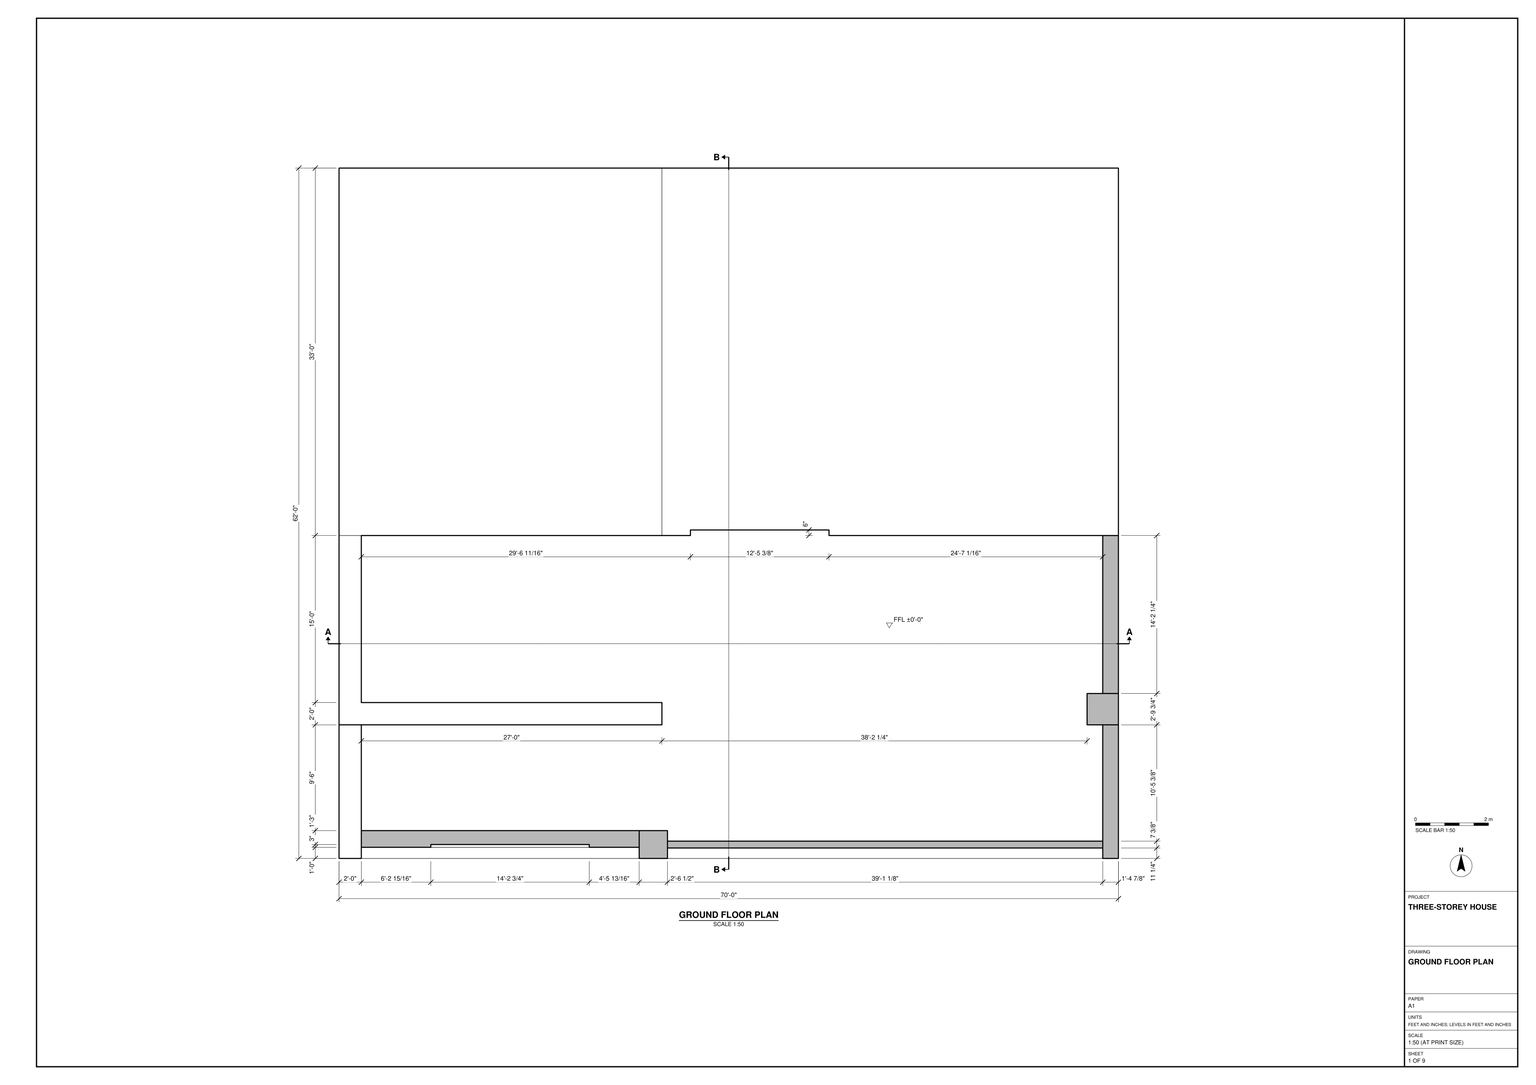
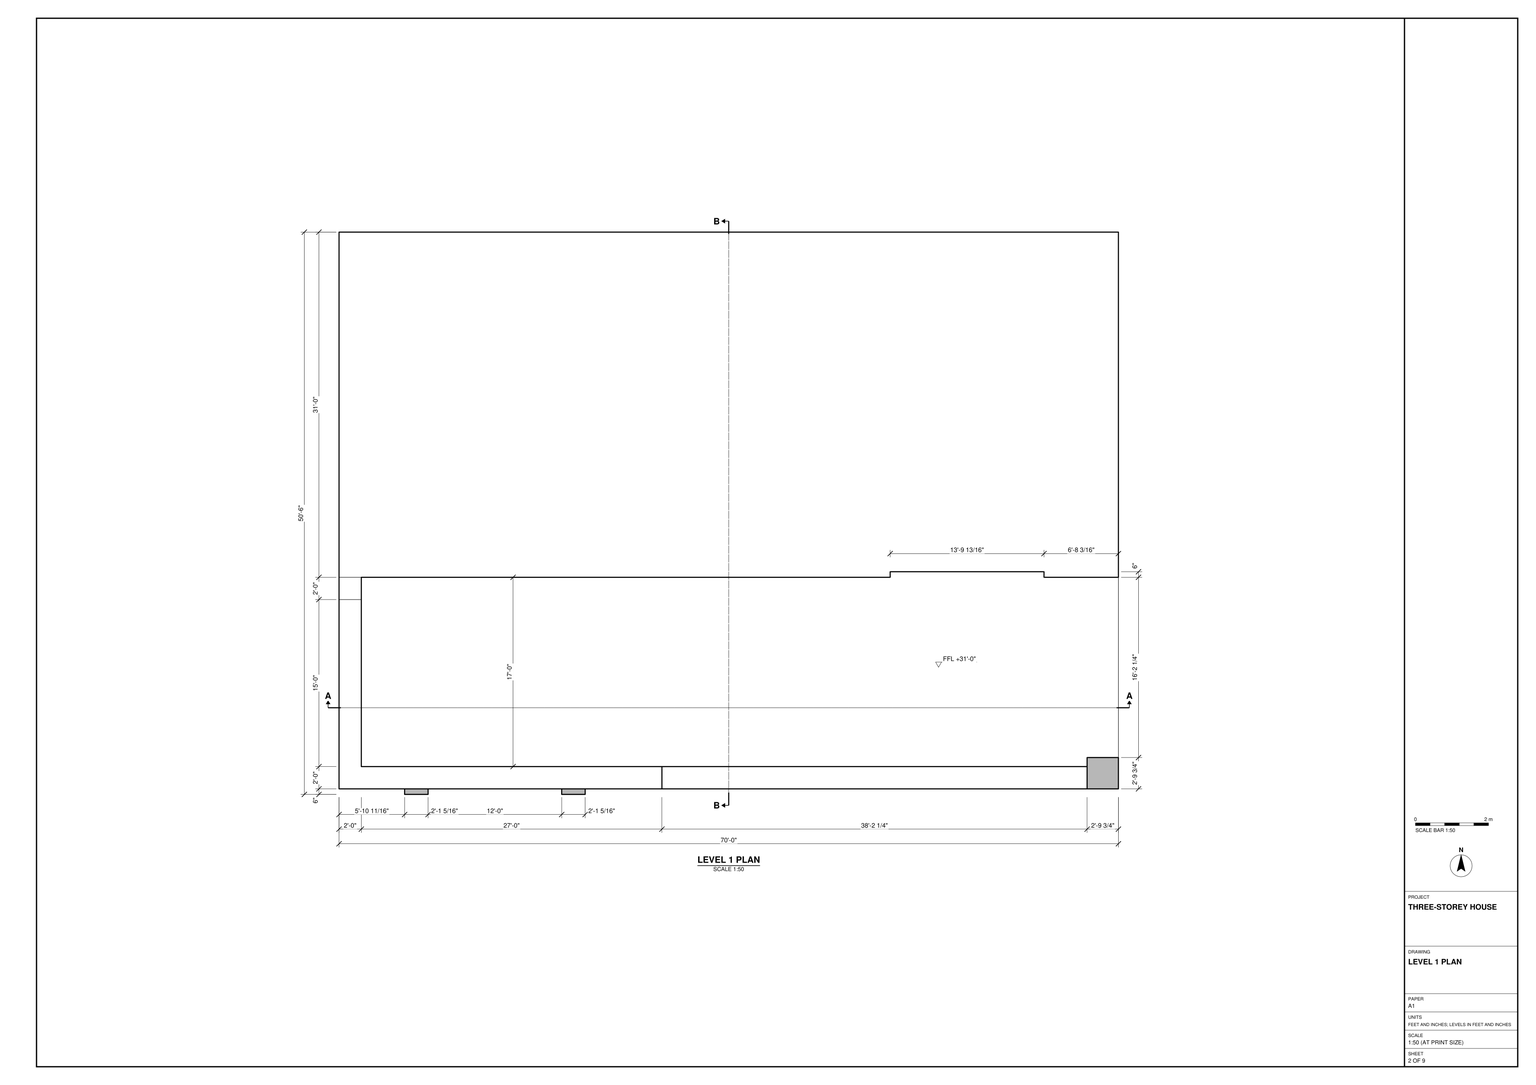
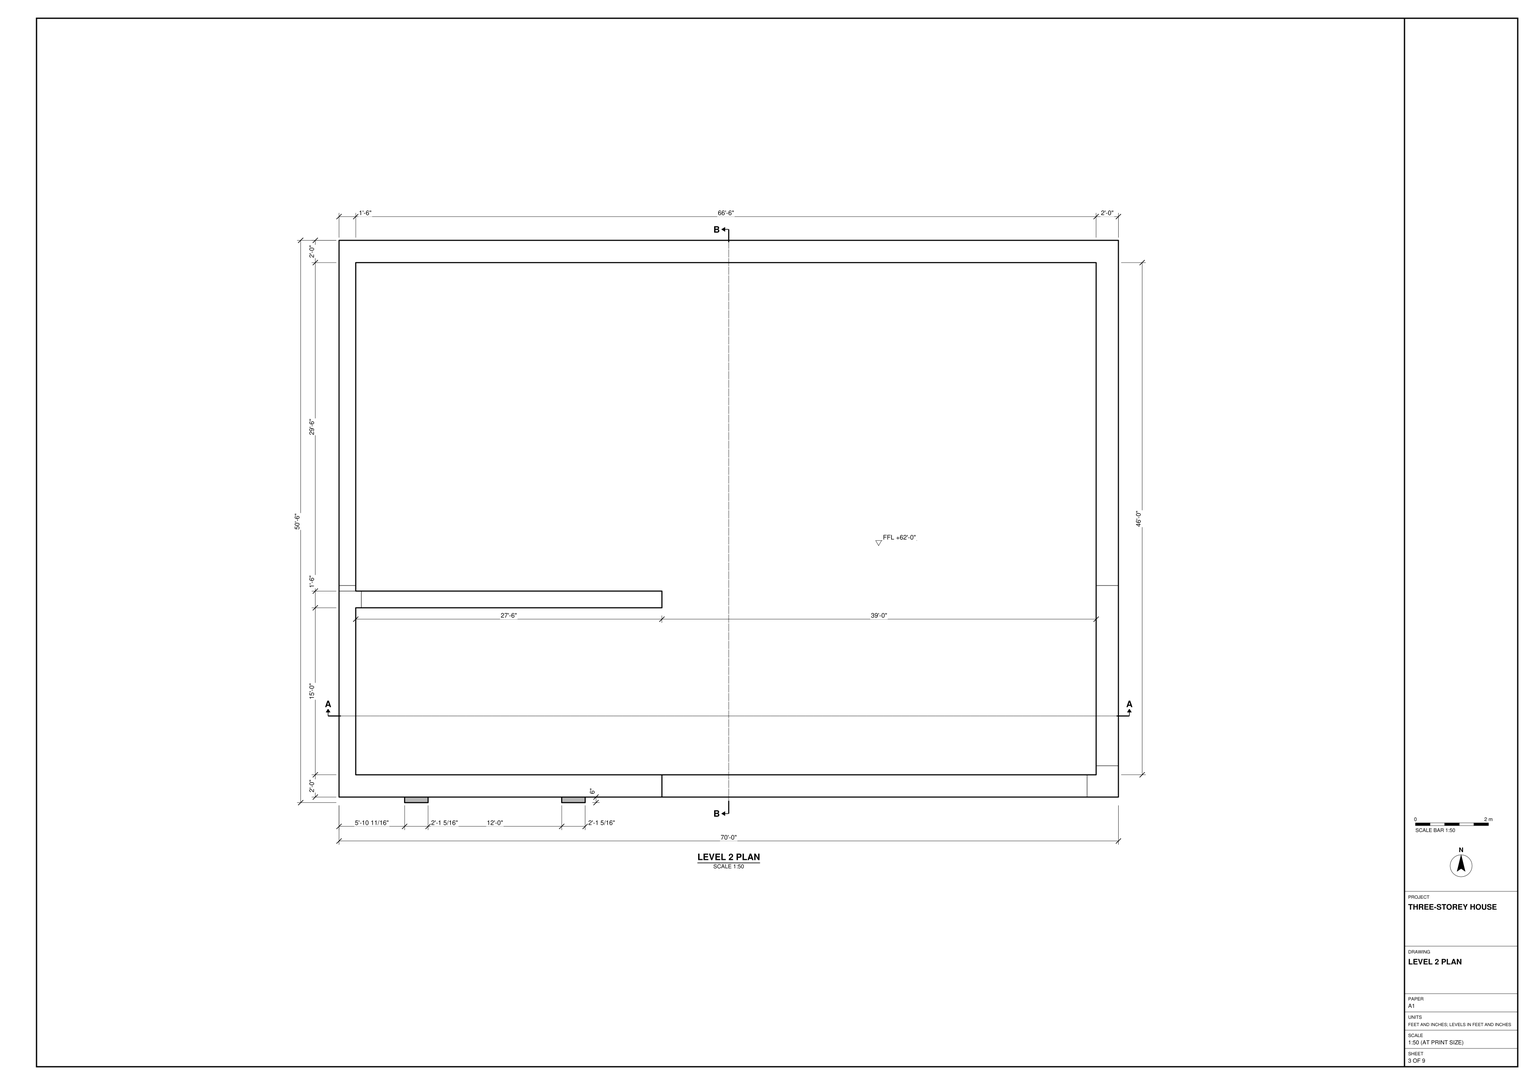
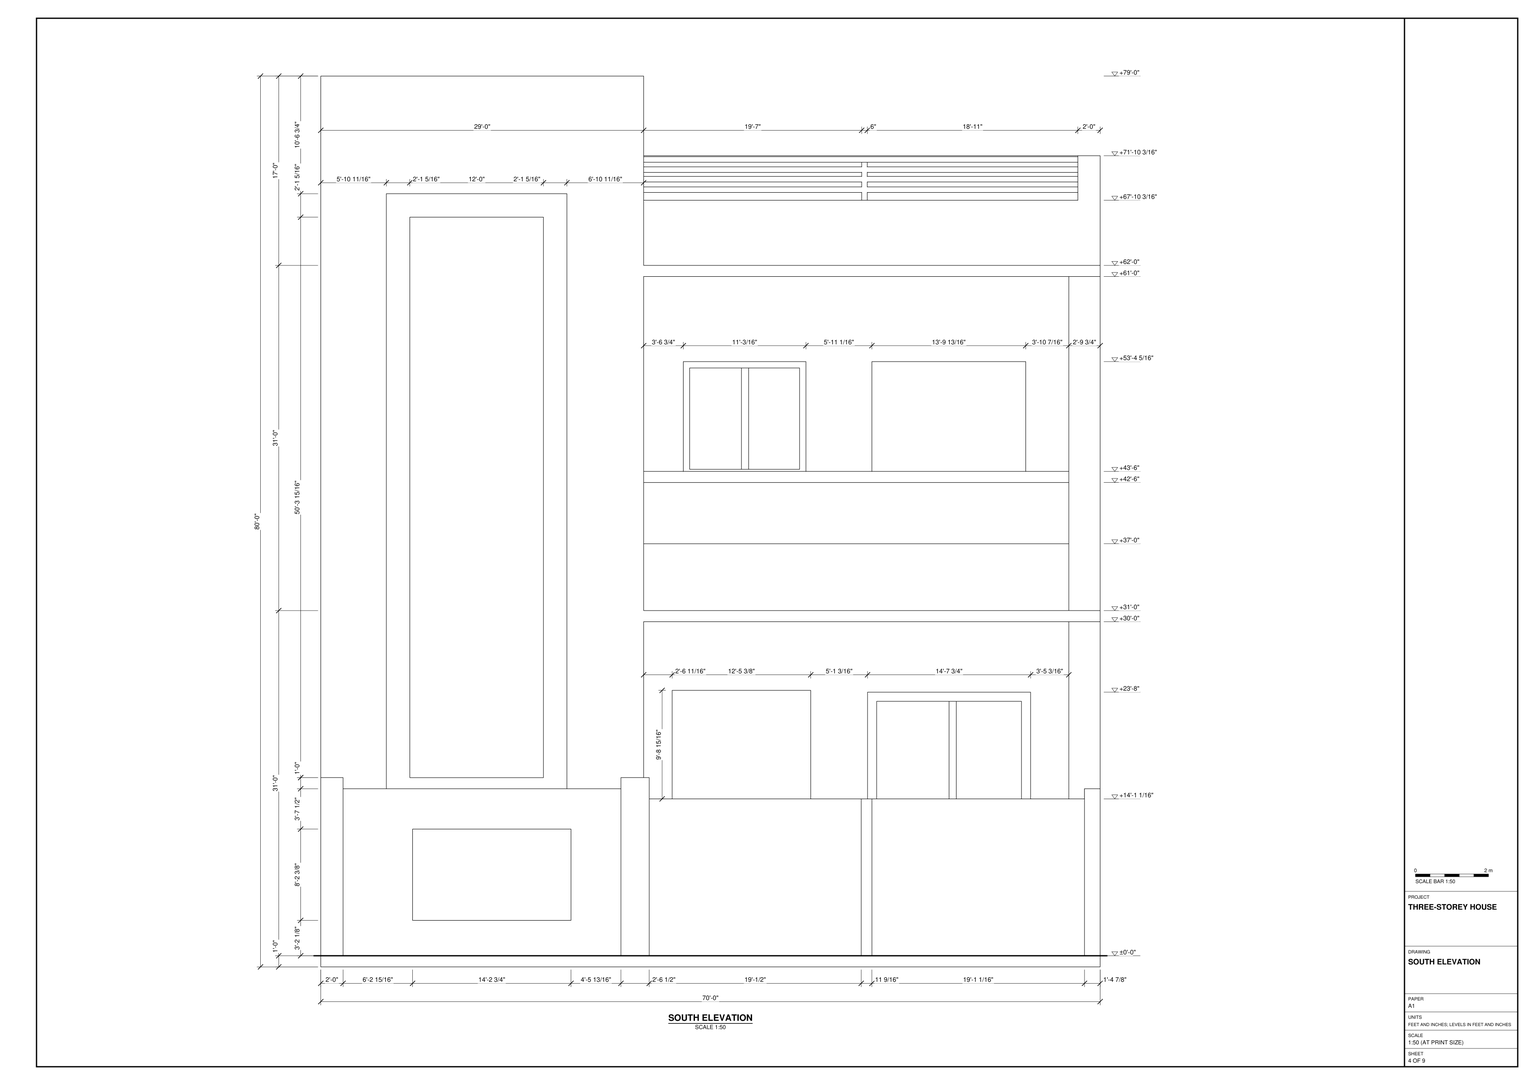
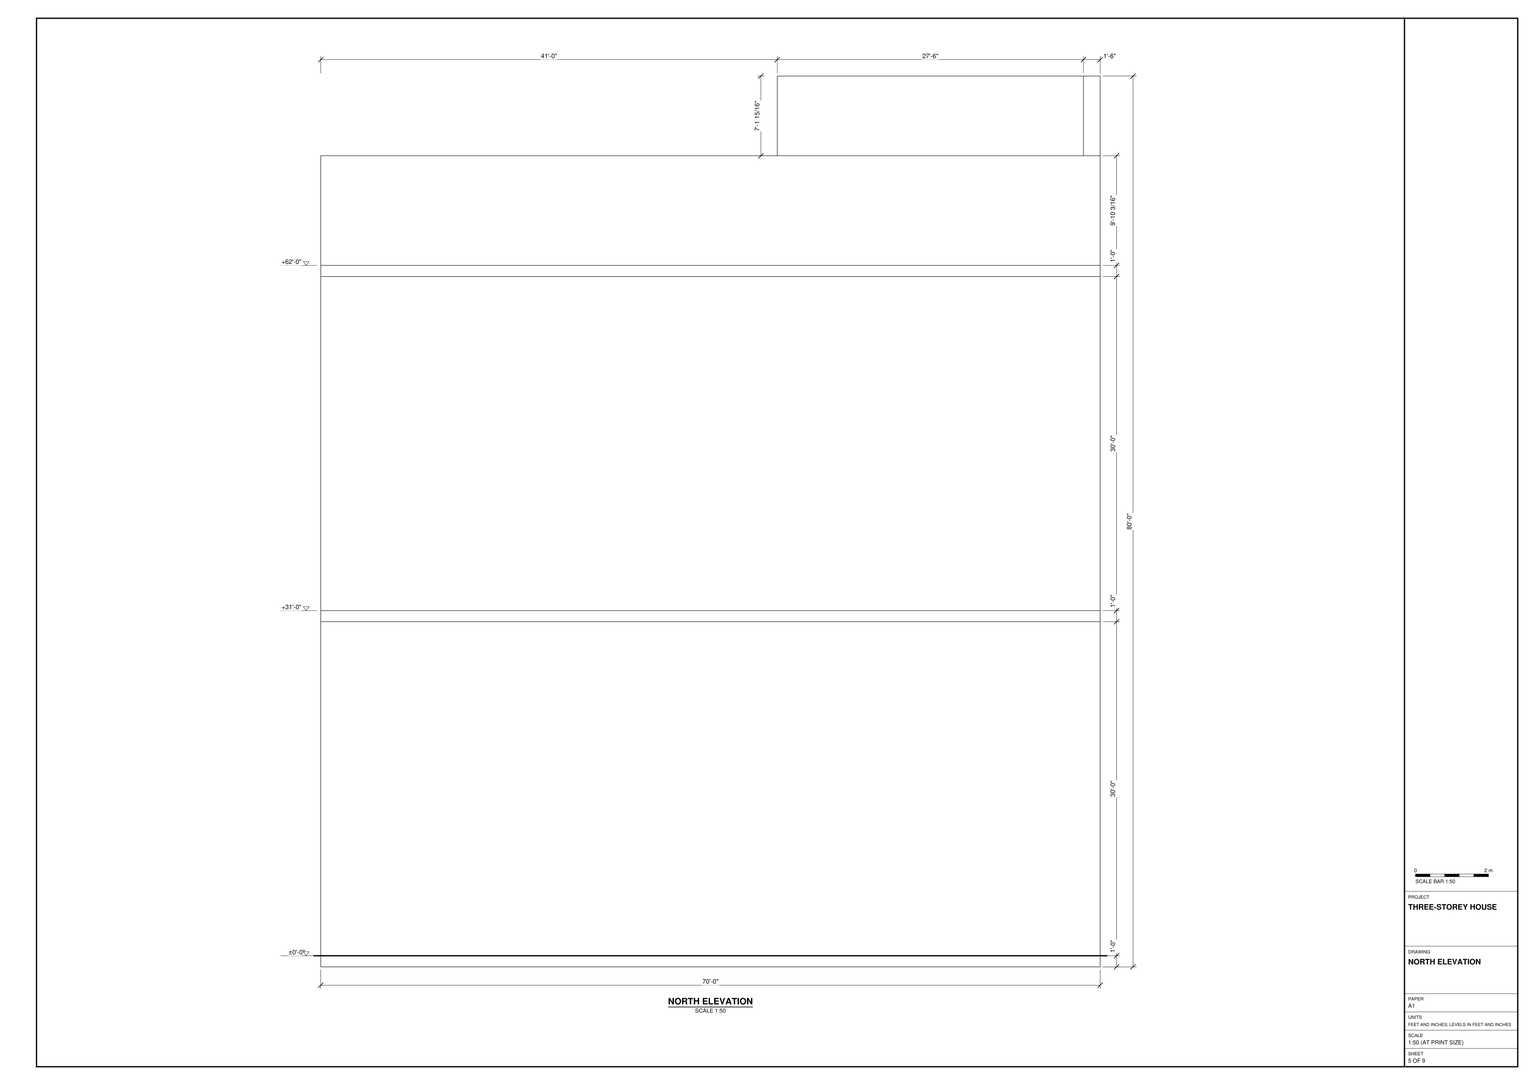
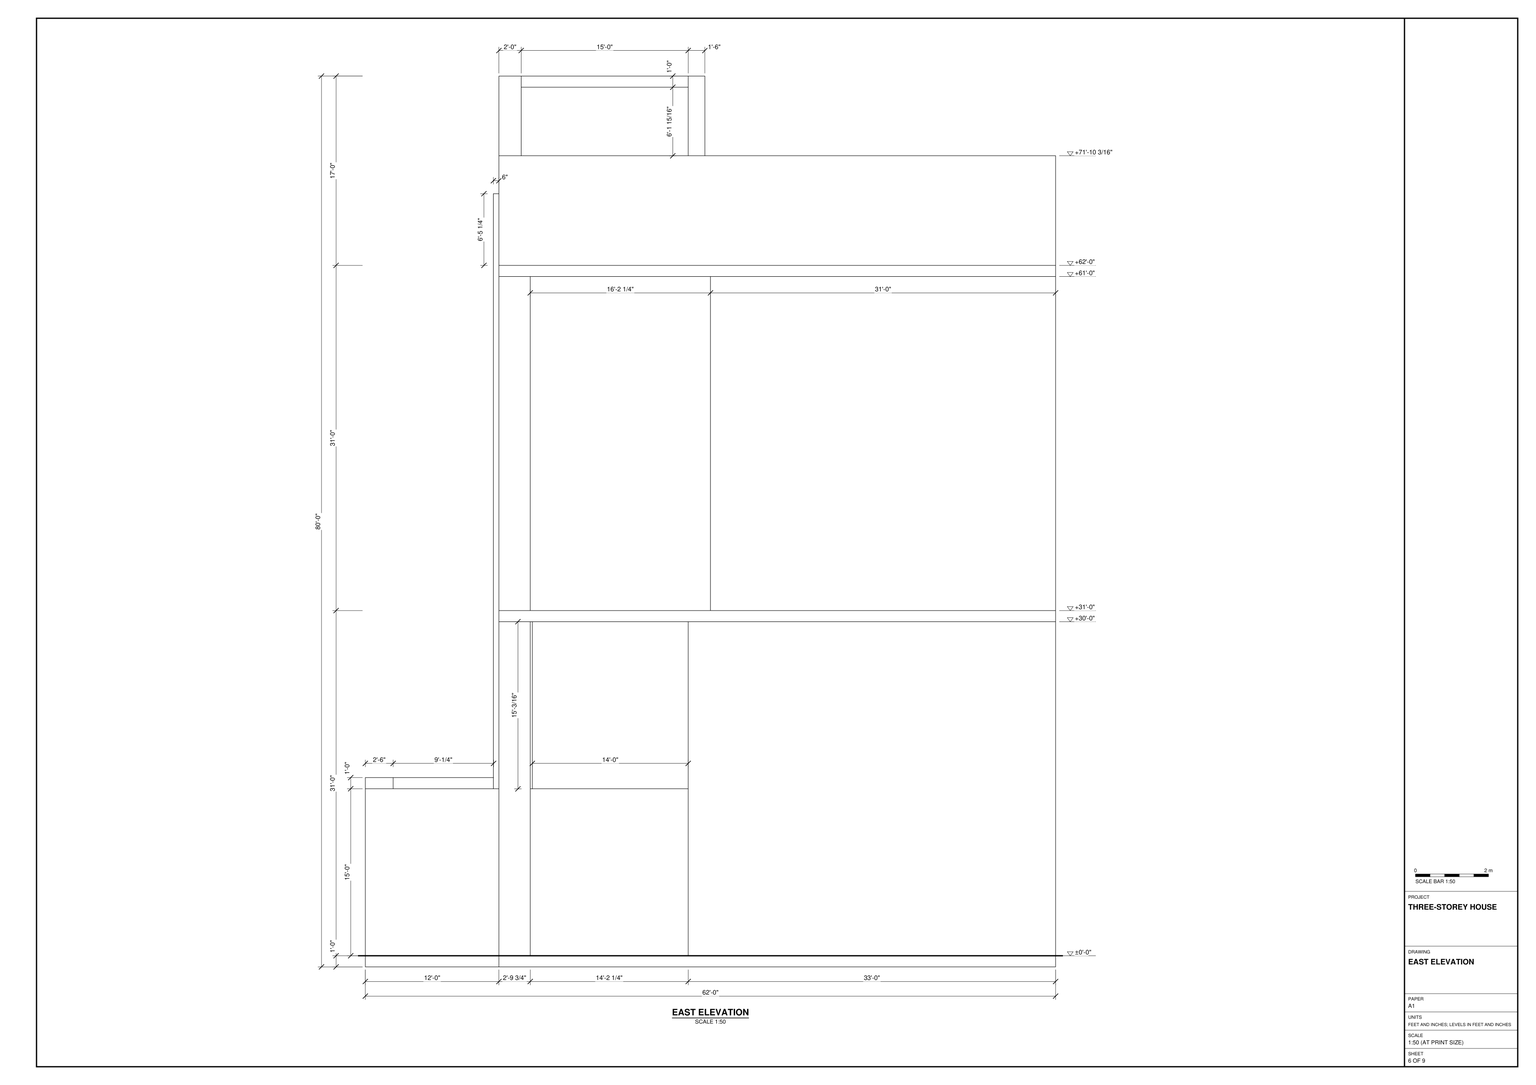
Build the three-storey house in SketchUp from task_files/diagram_01.pdf. Work in feet and inches. Set the overall width to 70'-0", the depth to 62'-0" and the height to 80'-0". Use ±0'-0" for the ground floor, +31'-0" for Level 1 and +62'-0" for Level 2.

Use the north arrow to align the plans. The upper floors retain the full width but stop short of the south edge of the ground floor. On the ground floor, follow the wall that turns inward from the west side, the projection on the east side and the changes in thickness along the south edge. Locate the shallow jogs in the ground-floor and Level 1 wall lines separately; they are not stacked above one another. At Level 2, follow the perimeter outline and the short wall extending east from its west side.

Use the sections and elevations to set slab edges, roof profiles and openings. Model walls at their drawn thicknesses, and include stairs, built-in joinery and main furniture where shown. Keep shell elements such as walls, slabs and roof in separate groups or components, do the same for each furniture or joinery piece, and use components for repeated parts. Decor and loose items may be any suitable library components. Save one SketchUp model as output_files/three_storey_house_with_recessed_upper_floors.skp.

# SketchUp Ruby script. Lengths in inches.
U = 1.inch
M = Sketchup.active_model
def pt(a) = Geom::Point3d.new(a.map { |v| v * U })
def face(e, loops, mat)
  f = e.add_face(loops[0].map { |a| pt(a) })
  loops[1..].each { |l| e.add_face(l.map { |a| pt(a) }).erase! }
  f.material = f.back_material = mat if mat
  f
end
# faces: each face lists its corners as indices into pts; further lists are holes
def faces(e, pts, list, mat = nil) = list.each { |f| face(e, (f[0].is_a?(Array) ? f : [f]).map { |l| l.map { |i| pts[i] } }, mat) }
# xy, xz, yz: faces in a plane at the given z, y or x. An outline is a flat list of corners, or four numbers for a rectangle; further outlines are holes
def ring(l) = l.size == 4 ? [[l[0], l[1]], [l[2], l[1]], [l[2], l[3]], [l[0], l[3]]] : l.each_slice(2).to_a
def flat(e, list, mat, &to3) = list.each { |f| face(e, (f[0].is_a?(Array) ? f : [f]).map { |l| ring(l).map { |u, v| to3.(u, v) } }, mat) }
def xy(e, z, list, mat = nil) = flat(e, list, mat) { |x, y| [x, y, z] }
def xz(e, y, list, mat = nil) = flat(e, list, mat) { |x, z| [x, y, z] }
def yz(e, x, list, mat = nil) = flat(e, list, mat) { |y, z| [x, y, z] }
def lines(e, pts, list) = list.each { |a, b| e.add_line(pt(pts[a]), pt(pts[b])) }
# prism: a flat outline (further loops are holes) pulled along v
def prism(e, loops, v, mat = nil)
  f = face(e, loops, mat); d = Geom::Vector3d.new(v.map { |x| x * U })
  f.pushpull(f.normal.samedirection?(d) ? d.length : -d.length)
end
def box(e, o, s, mat = nil) = prism(e, [[o, [o[0] + s[0], o[1], o[2]], [o[0] + s[0], o[1] + s[1], o[2]], [o[0], o[1] + s[1], o[2]]]], [0, 0, s[2]], mat)
def at(x, y, z, deg = 0) = Geom::Transformation.translation(pt([x, y, z])) * Geom::Transformation.rotation(ORIGIN, Z_AXIS, deg.degrees)
def axes(o, x, y, z) = Geom::Transformation.new([*x, 0, *y, 0, *z, 0, *pt(o).to_a, 1])
def part(name) = M.definitions.add(name)
# library, detail: a bought-in or finely detailed component or shape, given as its bounding box
def library(name, o, s) = part(name).tap { |d| box(d.entities, o, s) }
def detail(e, o, s) = box(e.add_group.entities, o, s)
def put(e, d, t, mat = nil) = e.add_instance(d, t).tap { |i| i.material = mat if mat }
def group(e, t, mat = nil) = e.add_group.tap { |g| g.transformation = t; g.material = mat if mat }.entities
root = M.entities
M.materials.add("[0018_Brown]").color = [96, 24, 24]
M.materials.add("[0027_PeachPuff]").color = [201, 172, 146]
M.materials.add("[0043_SaddleBrown]").color = [91, 45, 12]
M.materials.add("[0118_Thistle]").color = [216, 191, 216]
M.materials.add("[0136_Charcoal]").color = [35, 35, 35]
M.materials.add("[Beadboard]").color = [142, 93, 58]
M.materials.add("[Checker Plate]").color = [132, 132, 132]
M.materials.add("[Crushed Rock Gravel]").color = [173, 141, 102]
M.materials.add("[Stone Marble]").color = [143, 138, 136]
M.materials.add("[Translucent Glass Gray]").color = [128, 128, 128]
M.materials["[Translucent Glass Gray]"].alpha = 0.5
M.materials.add("[Wood Cherry Original]").color = [152, 86, 42]
M.materials.add("[Wood Floor]").color = [155, 105, 61]
xy(root,0,[[0,0,840,144],[0,144,840,744]])
xy(root,12,[[0,0,24,144],[323.51,0,354,30],[354,0,823.125,11.26],[823.125,0,840,144],[354,11.26,823.125,18.64],
  [24,12,323.51,30],[0,144,0,348,24,348,24,168,348,168,348,144],[806.25,144,840,177.75],[823.125,177.75,840,348],[0,348,348,744],
  [348,348,348,744,840,744,840,348,528.09,348,528.09,354,378.71,354,378.71,348]])
xy(root,12,[[24,0,323.51,12]],"[Crushed Rock Gravel]")
xy(root,12,[[354,18.64,823.125,18.64,823.125,144,806.25,144,806.25,177.75,823.125,177.75,823.125,348,528.09,348,528.09,354,378.71,354,378.71,348,24,348,24,168,348,168,348,144,24,144,24,30,354,30]],"[Stone Marble]")
xy(root,50.125,[[98.93,12,269.68,15]])
xy(root,148.5,[[98.93,12,269.68,15]])
xy(root,151.23,[[599.125,348,677.17,350],[684.94,348,755.22,350]])
xy(root,178.625,[[70.66,138,265.29,144]],"[0043_SaddleBrown]")
xy(root,181.0625,[[823.07,11.26,823.125,18.64]])
xy(root,181.0625,[[354,11.26,823.07,18.64]],"[0136_Charcoal]")
xy(root,192,[[823.125,0,840,144],[823.07,11.26,823.125,18.64],[823.125,177.75,840,348]])
xy(root,192,[[24,12,323.51,30]],"[Crushed Rock Gravel]")
xy(root,203.93,[[95.97,138,239.98,144]],"[0043_SaddleBrown]")
xy(root,204,[[0,0,24,144],[323.51,0,354,30]],"[Crushed Rock Gravel]")
xy(root,286.2,[[599.125,348,677.17,350],[684.94,348,755.22,350]])
xy(root,298,[[378.71,348,528.09,354]])
xy(root,372,[[433.85,198.0625,430.72,198.22,427.74,199.18,425.11,200.88,423.01,203.21,421.58,205.99,420.93,209.06,421.08,212.1875,422.04,215.17,423.75,217.8,426.07,219.9,428.86,221.33,431.92,221.98,435.05,221.83,438.03,220.87,440.66,219.16,442.76,216.84,444.19,214.05,444.85,210.99,444.69,207.86,443.73,204.88,442.03,202.25,439.7,200.15,436.92,198.72],[584.85,198.0625,581.72,198.22,578.74,199.18,576.11,200.88,574.01,203.21,572.58,205.99,571.93,209.06,572.08,212.1875,573.04,215.17,574.75,217.8,577.07,219.9,579.86,221.33,582.92,221.98,586.05,221.83,589.03,220.87,591.66,219.16,593.76,216.84,595.19,214.05,595.85,210.99,595.69,207.86,594.73,204.88,593.03,202.25,590.7,200.15,587.92,198.72],[748.17,198.0625,745.04,198.22,742.06,199.18,739.42,200.88,737.32,203.21,735.9,205.99,735.24,209.06,735.4,212.1875,736.36,215.17,738.06,217.8,740.38,219.9,743.17,221.33,746.23,221.98,749.36,221.83,752.34,220.87,754.97,219.16,757.07,216.84,758.5,214.05,759.16,210.99,759,207.86,758.04,204.88,756.34,202.25,754.02,200.15,751.23,198.72]])
xy(root,372,[[[348,144,348,168,24,168,24,348,840,348,840,177.75,806.25,177.75,806.25,144],[748.17,198.0625,751.23,198.72,754.02,200.15,756.34,202.25,758.04,204.88,759,207.86,759.16,210.99,758.5,214.05,757.07,216.84,754.97,219.16,752.34,220.87,749.36,221.83,746.23,221.98,743.17,221.33,740.38,219.9,738.06,217.8,736.36,215.17,735.4,212.1875,735.24,209.06,735.9,205.99,737.32,203.21,739.42,200.88,742.06,199.18,745.04,198.22],[584.85,198.0625,587.92,198.72,590.7,200.15,593.03,202.25,594.73,204.88,595.69,207.86,595.85,210.99,595.19,214.05,593.76,216.84,591.66,219.16,589.03,220.87,586.05,221.83,582.92,221.98,579.86,221.33,577.07,219.9,574.75,217.8,573.04,215.17,572.08,212.1875,571.93,209.06,572.58,205.99,574.01,203.21,576.11,200.88,578.74,199.18,581.72,198.22],[433.85,198.0625,436.92,198.72,439.7,200.15,442.03,202.25,443.73,204.88,444.69,207.86,444.85,210.99,444.19,214.05,442.76,216.84,440.66,219.16,438.03,220.87,435.05,221.83,431.92,221.98,428.86,221.33,426.07,219.9,423.75,217.8,422.04,215.17,421.08,212.1875,420.93,209.06,421.58,205.99,423.01,203.21,425.11,200.88,427.74,199.18,430.72,198.22]]],"[Wood Floor]")
xy(root,384,[[348,144,806.25,168],[806.25,144,840,177.75]])
xy(root,384,[[24,168,806.25,168,806.25,177.75,840,177.75,840,372,759.8125,372,759.8125,378,594,378,594,372,24,372]],"[Stone Marble]")
xy(root,456,[[348,144,806.25,154],[348,154,806.25,156],[348,156,806.25,168]])
xy(root,522,[[348,154,806.25,156]])
xy(root,536.21,[[397.58,372,453.39,374],[461.17,372,516.05,374]])
xy(root,645.43,[[397.58,372,453.39,374],[461.17,372,516.05,374]])
xy(root,652.29,[[594,372,759.8125,378]],"[Wood Cherry Original]")
xy(root,744,[[408.84,248.78,405.73,249.17,402.83,250.34,400.33,252.23,398.4,254.7,397.18,257.59,396.75,260.69,397.13,263.8,398.31,266.7,400.2,269.2,402.67,271.13,405.55,272.35,408.65,272.78,411.76,272.4,414.67,271.22,417.17,269.33,419.09,266.86,420.3125,263.98,420.75,260.87,420.36,257.76,419.18,254.86,417.3,252.36,414.83,250.44,411.94,249.21],[569.15,248.78,566.04,249.17,563.14,250.34,560.64,252.23,558.71,254.7,557.49,257.59,557.06,260.69,557.44,263.8,558.62,266.7,560.51,269.2,562.98,271.13,565.86,272.35,568.97,272.78,572.08,272.4,574.98,271.22,577.48,269.33,579.4,266.86,580.625,263.98,581.06,260.87,580.67,257.76,579.5,254.86,577.61,252.36,575.14,250.44,572.25,249.21],[722.4,248.78,719.29,249.17,716.39,250.34,713.89,252.23,711.96,254.7,710.74,257.59,710.31,260.69,710.69,263.8,711.87,266.7,713.76,269.2,716.23,271.13,719.11,272.35,722.22,272.78,725.33,272.4,728.23,271.22,730.73,269.33,732.65,266.86,733.875,263.98,734.31,260.87,733.92,257.76,732.75,254.86,730.86,252.36,728.39,250.44,725.5,249.21]])
xy(root,744,[[[348,144,348,168,24,168,24,372,840,372,840,177.75,806.25,177.75,806.25,144],[569.15,248.78,572.25,249.21,575.14,250.44,577.61,252.36,579.5,254.86,580.67,257.76,581.06,260.87,580.625,263.98,579.4,266.86,577.48,269.33,574.98,271.22,572.08,272.4,568.97,272.78,565.86,272.35,562.98,271.13,560.51,269.2,558.62,266.7,557.44,263.8,557.06,260.69,557.49,257.59,558.71,254.7,560.64,252.23,563.14,250.34,566.04,249.17],[722.4,248.78,725.5,249.21,728.39,250.44,730.86,252.36,732.75,254.86,733.92,257.76,734.31,260.87,733.875,263.98,732.65,266.86,730.73,269.33,728.23,271.22,725.33,272.4,722.22,272.78,719.11,272.35,716.23,271.13,713.76,269.2,711.87,266.7,710.69,263.8,710.31,260.69,710.74,257.59,711.96,254.7,713.89,252.23,716.39,250.34,719.29,249.17],[408.84,248.78,411.94,249.21,414.83,250.44,417.3,252.36,419.18,254.86,420.36,257.76,420.75,260.87,420.3125,263.98,419.09,266.86,417.17,269.33,414.67,271.22,411.76,272.4,408.65,272.78,405.55,272.35,402.67,271.13,400.2,269.2,398.31,266.7,397.13,263.8,396.75,260.69,397.18,257.59,398.4,254.7,400.33,252.23,402.83,250.34,405.73,249.17]]],"[Wood Floor]")
xy(root,756,[[18,168,816,168,816,720,18,720,18,366,348,366,348,348,18,348]])
xy(root,807.94,[[95.97,138,239.98,141],[95.97,141,239.98,144]])
xy(root,826.1875,[[[348,144,816,168],[585.98,152.98,585.21,153.08,584.48,153.38,583.86,153.86,583.39,154.48,583.09,155.2,582.98,155.98,583.09,156.75,583.39,157.48,583.86,158.1,584.48,158.58,585.21,158.875,585.98,158.98,586.76,158.875,587.48,158.58,588.11,158.1,588.58,157.48,588.88,156.75,588.98,155.98,588.88,155.2,588.58,154.48,588.11,153.86,587.48,153.38,586.76,153.08]],[585.98,152.98,585.21,153.08,584.48,153.38,583.86,153.86,583.39,154.48,583.09,155.2,582.98,155.98,583.09,156.75,583.39,157.48,583.86,158.1,584.48,158.58,585.21,158.875,585.98,158.98,586.76,158.875,587.48,158.58,588.11,158.1,588.58,157.48,588.88,156.75,588.98,155.98,588.88,155.2,588.58,154.48,588.11,153.86,587.48,153.38,586.76,153.08]])
xy(root,833.25,[[70.66,138,265.29,144]],"[0043_SaddleBrown]")
xy(root,867.15,[[585.98,152.98,586.76,153.08,587.48,153.38,588.11,153.86,588.58,154.48,588.88,155.2,588.98,155.98,588.88,156.75,588.58,157.48,588.11,158.1,587.48,158.58,586.76,158.875,585.98,158.98,585.21,158.875,584.48,158.58,583.86,158.1,583.39,157.48,583.09,156.75,582.98,155.98,583.09,155.2,583.39,154.48,583.86,153.86,584.48,153.38,585.21,153.08]])
xy(root,874.1875,[[816,144,840,144,840,744,0,744,0,366,18,366,18,720,816,720]])
xy(root,948,[[18,168,348,348]])
xy(root,960,[[0,144,348,144,348,168,18,168,18,348,348,348,348,366,0,366],[18,168,348,348]])
xz(root,0,[[0,0,840,12],[0,12,24,204],[323.51,12,354,204],[823.125,12,840,192]],"[Crushed Rock Gravel]")
xz(root,11.26,[[823.07,181.0625,823.125,192]])
xz(root,11.26,[[582.48,12,594.05,181.0625]],"[0136_Charcoal]")
xz(root,11.26,[[354,12,582.48,181.0625],[594.05,12,823.125,181.0625]],"[Beadboard]")
xz(root,12,[[[24,12,323.51,192],[98.93,50.125,269.68,148.5]]],"[Crushed Rock Gravel]")
xz(root,15,[[98.93,50.125,269.68,148.5]])
xz(root,18.64,[[823.07,181.0625,823.125,192]])
xz(root,18.64,[[354,12,823.125,181.0625]],"[Beadboard]")
xz(root,30,[[24,12,323.51,192],[323.51,12,354,204]])
xz(root,138,[[[70.66,178.625,265.29,833.25],[95.97,203.93,239.98,807.94]]],"[0043_SaddleBrown]")
xz(root,144,[[0,12,24,204],[823.125,12,840,192],[[70.66,178.625,265.29,833.25],[95.97,203.93,239.98,807.94]]])
xz(root,144,[[806.25,12,823.125,12,823.125,192,840,192,840,372,806.25,372],[348,384,806.25,456],[806.25,384,840,744],[348,756,840,756,840,874.1875,816,874.1875,816,826.1875,348,826.1875]],"[0118_Thistle]")
xz(root,144,[[[24,12,348,12,348,372,840,372,840,384,348,384,348,744,840,744,840,756,348,756,348,960,0,960,0,204,24,204],[70.66,178.625,265.29,833.25]]],"[Checker Plate]")
xz(root,144,[[95.97,203.93,239.98,807.94]],"[Translucent Glass Gray]")
xz(root,154,[[348,456,806.25,522]],"[Translucent Glass Gray]")
xz(root,156,[[348,456,806.25,522]],"[Translucent Glass Gray]")
xz(root,168,[[24,12,348,372],[24,384,348,744],[348,384,806.25,456],[18,756,348,948],[348,756,816,826.1875],
  [18,948,348,960]])
xz(root,177.75,[[806.25,12,806.25,372,840,372,840,192,823.125,192,823.125,12],[823.125,12,840,192],[806.25,384,840,744]])
xz(root,348,[[823.125,12,840,192],[18,756,348,948],[18,948,348,960]])
xz(root,348,[[[24,12,378.71,12,378.71,298,528.09,298,528.09,12,823.125,12,823.125,192,840,192,840,372,24,372],[589.3,141.4,765.05,296.03]]],"[0027_PeachPuff]")
xz(root,348,[[[589.3,141.4,765.05,296.03],[599.125,151.23,755.22,286.2]],[677.17,151.23,684.94,286.2]],"[0136_Charcoal]")
xz(root,350,[[599.125,151.23,677.17,286.2],[684.94,151.23,755.22,286.2]],"[Translucent Glass Gray]")
xz(root,354,[[378.71,12,528.09,298]],"[0018_Brown]")
xz(root,366,[[18,756,348,960],[0,874.1875,18,960]])
xz(root,372,[[[24,384,594,384,594,652.29,759.8125,652.29,759.8125,384,840,384,840,744,24,744],[390.72,529.35,522.91,652.29]]],"[0027_PeachPuff]")
xz(root,372,[[[390.72,529.35,522.91,652.29],[397.58,536.21,516.05,645.43]],[453.39,536.21,461.17,645.43]],"[0136_Charcoal]")
xz(root,374,[[397.58,536.21,453.39,645.43],[461.17,536.21,516.05,645.43]],"[Translucent Glass Gray]")
xz(root,378,[[594,384,759.8125,652.29]],"[Wood Cherry Original]")
xz(root,720,[[18,756,816,874.1875]])
xz(root,744,[[0,0,840,12],[0,12,840,372],[0,372,840,384],[0,384,840,744],[0,744,840,756],
  [0,756,840,874.1875]])
yz(root,0,[[0,0,144,12],[144,0,744,12],[144,12,144,960,366,960,366,874.1875,744,874.1875,744,12]])
yz(root,0,[[0,12,144,204]],"[Crushed Rock Gravel]")
yz(root,18,[[168,756,348,948],[366,756,720,874.1875],[168,948,348,960]])
yz(root,24,[[12,12,30,192],[168,12,180,372],[180,12,348,372],[168,384,372,744]])
yz(root,24,[[0,12,12,12,12,192,30,192,30,12,144,12,144,204,0,204]],"[Crushed Rock Gravel]")
yz(root,70.66,[[138,178.625,144,833.25]],"[0043_SaddleBrown]")
yz(root,95.97,[[138,203.93,144,807.94]],"[0043_SaddleBrown]")
yz(root,98.93,[[12,50.125,15,148.5]])
yz(root,239.98,[[138,203.93,144,807.94]],"[0043_SaddleBrown]")
yz(root,265.29,[[138,178.625,144,833.25]],"[0043_SaddleBrown]")
yz(root,269.68,[[12,50.125,15,148.5]])
yz(root,323.51,[[12,12,30,192]])
yz(root,323.51,[[0,12,12,204],[12,192,30,204]],"[Crushed Rock Gravel]")
yz(root,348,[[144,12,168,372],[144,384,168,456],[144,456,154,456,154,522,156,522,155.37,522.03,154.75,522.13,154.15,522.29,153.56,522.52,153,522.8,152.47,523.15,151.99,523.54,151.54,523.99,151.15,524.47,150.8,525,150.52,525.56,150.29,526.15,150.13,526.75,150.03,527.37,150,528,150.03,528.63,150.13,529.25,150.29,529.85,150.52,530.44,150.8,531,151.15,531.53,151.54,532.01,151.99,532.46,152.47,532.85,153,533.2,153.56,533.48,154.15,533.71,154.75,533.87,155.37,533.97,156,534,156.63,533.97,157.25,533.87,157.85,533.71,158.44,533.48,159,533.2,159.53,532.85,160.01,532.46,160.46,532.01,160.85,531.53,161.2,531,161.48,530.44,161.71,529.85,161.87,529.25,161.97,528.63,162,528,161.97,527.37,161.87,526.75,161.71,526.15,161.48,525.56,161.2,525,160.85,524.47,160.46,523.99,160.01,523.54,159.53,523.15,159,522.8,158.44,522.52,157.85,522.29,157.25,522.13,156.63,522.03,156,522,156,456,168,456,168,744,144,744],[154,456,156,521.9375],[154,521.9375,156,522],
  [144,756,168,826.1875],[348,756,366,960],[[144,826.1875,168,960],[156,834.58,155.22,834.6875,154.5,834.99,153.88,835.46,153.4,836.08,153.1,836.81,153,837.58,153.1,838.36,153.4,839.08,153.88,839.7,154.5,840.18,155.22,840.48,156,840.58,156.78,840.48,157.5,840.18,158.12,839.7,158.6,839.08,158.9,838.36,159,837.58,158.9,836.81,158.6,836.08,158.12,835.46,157.5,834.99,156.78,834.6875],[156,845.9,155.22,846,154.5,846.3,153.88,846.77,153.4,847.4,153.1,848.12,153,848.9,153.1,849.67,153.4,850.4,153.88,851.02,154.5,851.49,155.22,851.79,156,851.9,156.78,851.79,157.5,851.49,158.12,851.02,158.6,850.4,158.9,849.67,159,848.9,158.9,848.12,158.6,847.4,158.12,846.77,157.5,846.3,156.78,846],[156,856.21,155.22,856.3125,154.5,856.61,153.88,857.09,153.4,857.71,153.1,858.43,153,859.21,153.1,859.99,153.4,860.71,153.88,861.33,154.5,861.81,155.22,862.11,156,862.21,156.78,862.11,157.5,861.81,158.12,861.33,158.6,860.71,158.9,859.99,159,859.21,158.9,858.43,158.6,857.71,158.12,857.09,157.5,856.61,156.78,856.3125],[156,867.15,155.22,867.25,154.5,867.55,153.88,868.02,153.4,868.65,153.1,869.37,153,870.15,153.1,870.92,153.4,871.65,153.88,872.27,154.5,872.74,155.22,873.04,156,873.15,156.78,873.04,157.5,872.74,158.12,872.27,158.6,871.65,158.9,870.92,159,870.15,158.9,869.37,158.6,868.65,158.12,868.02,157.5,867.55,156.78,867.25]],[168,948,348,960]])
yz(root,354,[[0,12,11.26,12,11.26,181.0625,18.64,181.0625,18.64,12,30,12,30,204,0,204],[11.26,12,18.64,181.0625]])
yz(root,378.71,[[348,12,354,298]])
yz(root,397.58,[[372,536.21,374,645.43]])
yz(root,453.39,[[372,536.21,374,645.43]])
yz(root,461.17,[[372,536.21,374,645.43]])
yz(root,516.05,[[372,536.21,374,645.43]])
yz(root,528.09,[[348,12,354,298]])
yz(root,594,[[372,384,378,652.29]],"[Wood Cherry Original]")
yz(root,599.125,[[348,151.23,350,286.2]])
yz(root,677.17,[[348,151.23,350,286.2]])
yz(root,684.94,[[348,151.23,350,286.2]])
yz(root,755.22,[[348,151.23,350,286.2]])
yz(root,759.8125,[[372,384,378,652.29]],"[Wood Cherry Original]")
yz(root,806.25,[[144,12,177.75,372],[144,384,168,456],[168,384,168,456,156,456,156,522,156.63,522.03,157.25,522.13,157.85,522.29,158.44,522.52,159,522.8,159.53,523.15,160.01,523.54,160.46,523.99,160.85,524.47,161.2,525,161.48,525.56,161.71,526.15,161.87,526.75,161.97,527.37,162,528,161.97,528.63,161.87,529.25,161.71,529.85,161.48,530.44,161.2,531,160.85,531.53,160.46,532.01,160.01,532.46,159.53,532.85,159,533.2,158.44,533.48,157.85,533.71,157.25,533.87,156.63,533.97,156,534,155.37,533.97,154.75,533.87,154.15,533.71,153.56,533.48,153,533.2,152.47,532.85,151.99,532.46,151.54,532.01,151.15,531.53,150.8,531,150.52,530.44,150.29,529.85,150.13,529.25,150.03,528.63,150,528,150.03,527.37,150.13,526.75,150.29,526.15,150.52,525.56,150.8,525,151.15,524.47,151.54,523.99,151.99,523.54,152.47,523.15,153,522.8,153.56,522.52,154.15,522.29,154.75,522.13,155.37,522.03,156,522,154,522,154,456,144,456,144,744,177.75,744,177.75,384],[154,456,156,522],[156,522,156.63,522.03,157.25,522.13,157.85,522.29,158.44,522.52,159,522.8,159.53,523.15,160.01,523.54,160.46,523.99,160.85,524.47,161.2,525,161.48,525.56,161.71,526.15,161.87,526.75,161.97,527.37,162,528,161.97,528.63,161.87,529.25,161.71,529.85,161.48,530.44,161.2,531,160.85,531.53,160.46,532.01,160.01,532.46,159.53,532.85,159,533.2,158.44,533.48,157.85,533.71,157.25,533.87,156.63,533.97,156,534,155.37,533.97,154.75,533.87,154.15,533.71,153.56,533.48,153,533.2,152.47,532.85,151.99,532.46,151.54,532.01,151.15,531.53,150.8,531,150.52,530.44,150.29,529.85,150.13,529.25,150.03,528.63,150,528,150.03,527.37,150.13,526.75,150.29,526.15,150.52,525.56,150.8,525,151.15,524.47,151.54,523.99,151.99,523.54,152.47,523.15,153,522.8,153.56,522.52,154.15,522.29,154.75,522.13,155.37,522.03]])
yz(root,816,[[[168,756,168,826.1875,144,826.1875,144,874.1875,720,874.1875,720,756],[156,845.9,156.78,846,157.5,846.3,158.12,846.77,158.6,847.4,158.9,848.12,159,848.9,158.9,849.67,158.6,850.4,158.12,851.02,157.5,851.49,156.78,851.79,156,851.9,155.22,851.79,154.5,851.49,153.88,851.02,153.4,850.4,153.1,849.67,153,848.9,153.1,848.12,153.4,847.4,153.88,846.77,154.5,846.3,155.22,846],[156,856.21,156.78,856.3125,157.5,856.61,158.12,857.09,158.6,857.71,158.9,858.43,159,859.21,158.9,859.99,158.6,860.71,158.12,861.33,157.5,861.81,156.78,862.11,156,862.21,155.22,862.11,154.5,861.81,153.88,861.33,153.4,860.71,153.1,859.99,153,859.21,153.1,858.43,153.4,857.71,153.88,857.09,154.5,856.61,155.22,856.3125],[156,867.15,156.78,867.25,157.5,867.55,158.12,868.02,158.6,868.65,158.9,869.37,159,870.15,158.9,870.92,158.6,871.65,158.12,872.27,157.5,872.74,156.78,873.04,156,873.15,155.22,873.04,154.5,872.74,153.88,872.27,153.4,871.65,153.1,870.92,153,870.15,153.1,869.37,153.4,868.65,153.88,868.02,154.5,867.55,155.22,867.25],[156,834.58,156.78,834.6875,157.5,834.99,158.12,835.46,158.6,836.08,158.9,836.81,159,837.58,158.9,838.36,158.6,839.08,158.12,839.7,157.5,840.18,156.78,840.48,156,840.58,155.22,840.48,154.5,840.18,153.88,839.7,153.4,839.08,153.1,838.36,153,837.58,153.1,836.81,153.4,836.08,153.88,835.46,154.5,834.99,155.22,834.6875]],[156,834.58,156.78,834.6875,157.5,834.99,158.12,835.46,158.6,836.08,158.9,836.81,159,837.58,158.9,838.36,158.6,839.08,158.12,839.7,157.5,840.18,156.78,840.48,156,840.58,155.22,840.48,154.5,840.18,153.88,839.7,153.4,839.08,153.1,838.36,153,837.58,153.1,836.81,153.4,836.08,153.88,835.46,154.5,834.99,155.22,834.6875],[156,845.9,156.78,846,157.5,846.3,158.12,846.77,158.6,847.4,158.9,848.12,159,848.9,158.9,849.67,158.6,850.4,158.12,851.02,157.5,851.49,156.78,851.79,156,851.9,155.22,851.79,154.5,851.49,153.88,851.02,153.4,850.4,153.1,849.67,153,848.9,153.1,848.12,153.4,847.4,153.88,846.77,154.5,846.3,155.22,846],[156,856.21,156.78,856.3125,157.5,856.61,158.12,857.09,158.6,857.71,158.9,858.43,159,859.21,158.9,859.99,158.6,860.71,158.12,861.33,157.5,861.81,156.78,862.11,156,862.21,155.22,862.11,154.5,861.81,153.88,861.33,153.4,860.71,153.1,859.99,153,859.21,153.1,858.43,153.4,857.71,153.88,857.09,154.5,856.61,155.22,856.3125],[156,867.15,156.78,867.25,157.5,867.55,158.12,868.02,158.6,868.65,158.9,869.37,159,870.15,158.9,870.92,158.6,871.65,158.12,872.27,157.5,872.74,156.78,873.04,156,873.15,155.22,873.04,154.5,872.74,153.88,872.27,153.4,871.65,153.1,870.92,153,870.15,153.1,869.37,153.4,868.65,153.88,868.02,154.5,867.55,155.22,867.25]])
yz(root,823.07,[[11.26,181.0625,18.64,192]])
yz(root,823.125,[[0,12,11.26,192],[11.26,12,18.64,181.0625],[18.64,12,144,192],[177.75,12,348,192],[11.26,181.0625,18.64,192]])
yz(root,840,[[144,0,744,12],[348,12,744,372],[144,372,744,384],[144,384,177.75,744],[372,384,744,744],
  [144,744,744,756],[144,756,744,874.1875]])
yz(root,840,[[0,0,144,12],[0,12,144,192],[144,12,177.75,372],[177.75,12,348,192]],"[Crushed Rock Gravel]")
p = [[806.25,155.37,522.03],[806.25,154.75,522.13],[348,154.75,522.13],[348,155.37,522.03],[806.25,156,522],[348,156,522],
  [806.25,156.63,522.03],[348,156.63,522.03],[806.25,157.25,522.13],[348,157.25,522.13],[806.25,154.15,522.29],[348,154.15,522.29],
  [806.25,157.85,522.29],[348,157.85,522.29],[806.25,153.56,522.52],[348,153.56,522.52],[806.25,158.44,522.52],[348,158.44,522.52],
  [806.25,153,522.8],[348,153,522.8],[806.25,159,522.8],[348,159,522.8],[806.25,152.47,523.15],[348,152.47,523.15],
  [806.25,159.53,523.15],[348,159.53,523.15],[806.25,151.99,523.54],[348,151.99,523.54],[806.25,160.01,523.54],[348,160.01,523.54],
  [806.25,151.54,523.99],[348,151.54,523.99],[806.25,160.46,523.99],[348,160.46,523.99],[806.25,151.15,524.47],[348,151.15,524.47],
  [806.25,160.85,524.47],[348,160.85,524.47],[806.25,150.8,525],[348,150.8,525],[806.25,161.2,525],[348,161.2,525],
  [806.25,150.52,525.56],[348,150.52,525.56],[806.25,161.48,525.56],[348,161.48,525.56],[806.25,150.29,526.15],[348,150.29,526.15],
  [806.25,161.71,526.15],[348,161.71,526.15],[806.25,150.13,526.75],[348,150.13,526.75],[806.25,161.87,526.75],[348,161.87,526.75],
  [806.25,150.03,527.37],[348,150.03,527.37],[806.25,161.97,527.37],[348,161.97,527.37],[806.25,150,528],[348,150,528],
  [806.25,162,528],[348,162,528],[806.25,150.03,528.63],[348,150.03,528.63],[806.25,161.97,528.63],[348,161.97,528.63],
  [806.25,150.13,529.25],[348,150.13,529.25],[806.25,161.87,529.25],[348,161.87,529.25],[806.25,150.29,529.85],[348,150.29,529.85],
  [806.25,161.71,529.85],[348,161.71,529.85],[806.25,150.52,530.44],[348,150.52,530.44],[806.25,161.48,530.44],[348,161.48,530.44],
  [806.25,150.8,531],[348,150.8,531],[806.25,161.2,531],[348,161.2,531],[806.25,151.15,531.53],[348,151.15,531.53],
  [806.25,160.85,531.53],[348,160.85,531.53],[806.25,151.54,532.01],[348,151.54,532.01],[806.25,160.46,532.01],[348,160.46,532.01],
  [806.25,151.99,532.46],[348,151.99,532.46],[806.25,160.01,532.46],[348,160.01,532.46],[806.25,152.47,532.85],[348,152.47,532.85],
  [806.25,159.53,532.85],[348,159.53,532.85],[806.25,153,533.2],[348,153,533.2],[806.25,159,533.2],[348,159,533.2],
  [806.25,153.56,533.48],[348,153.56,533.48],[806.25,158.44,533.48],[348,158.44,533.48],[806.25,154.15,533.71],[348,154.15,533.71],
  [806.25,157.85,533.71],[348,157.85,533.71],[806.25,154.75,533.87],[348,154.75,533.87],[806.25,157.25,533.87],[348,157.25,533.87],
  [806.25,155.37,533.97],[348,155.37,533.97],[806.25,156.63,533.97],[348,156.63,533.97],[806.25,156,534],[348,156,534],
  [585.21,153.08,826.1875],[585.98,152.98,826.1875],[585.98,152.98,855.48],[585.98,152.98,867.15],[585.21,153.08,867.15],[585.21,153.08,855.48],
  [586.76,153.08,826.1875],[586.76,153.08,855.48],[586.76,153.08,867.15],[584.48,153.38,826.1875],[584.48,153.38,867.15],[584.48,153.38,855.48],
  [587.48,153.38,826.1875],[587.48,153.38,855.48],[587.48,153.38,867.15],[583.86,153.86,826.1875],[583.86,153.86,867.15],[583.86,153.86,855.48],
  [588.11,153.86,826.1875],[588.11,153.86,855.48],[588.11,153.86,867.15],[583.39,154.48,826.1875],[583.39,154.48,867.15],[583.39,154.48,855.48],
  [588.58,154.48,826.1875],[588.58,154.48,855.48],[588.58,154.48,867.15],[583.09,155.2,826.1875],[583.09,155.2,867.15],[583.09,155.2,855.48],
  [588.88,155.2,826.1875],[588.88,155.2,855.48],[588.88,155.2,867.15],[582.98,155.98,867.15],[582.98,155.98,855.48],[582.98,155.98,826.1875],
  [588.98,155.98,826.1875],[588.98,155.98,855.48],[588.98,155.98,867.15],[583.09,156.75,867.15],[583.09,156.75,855.48],[583.09,156.75,826.1875],
  [588.88,156.75,826.1875],[588.88,156.75,855.48],[588.88,156.75,867.15],[583.39,157.48,867.15],[583.39,157.48,855.48],[583.39,157.48,826.1875],
  [588.58,157.48,826.1875],[588.58,157.48,855.48],[588.58,157.48,867.15],[583.86,158.1,867.15],[583.86,158.1,855.48],[583.86,158.1,826.1875],
  [588.11,158.1,826.1875],[588.11,158.1,855.48],[588.11,158.1,867.15],[584.48,158.58,867.15],[584.48,158.58,855.48],[584.48,158.58,826.1875],
  [587.48,158.58,826.1875],[587.48,158.58,855.48],[587.48,158.58,867.15],[585.21,158.875,867.15],[585.21,158.875,855.48],[585.21,158.875,826.1875],
  [586.76,158.875,855.48],[586.76,158.875,867.15],[586.76,158.875,826.1875],[585.98,158.98,867.15],[585.98,158.98,855.48],[585.98,158.98,826.1875],
  [816,156,834.58],[816,155.22,834.6875],[348,155.22,834.6875],[348,156,834.58],[816,156.78,834.6875],[348,156.78,834.6875],
  [816,154.5,834.99],[348,154.5,834.99],[816,157.5,834.99],[348,157.5,834.99],[816,153.88,835.46],[348,153.88,835.46],
  [816,158.12,835.46],[348,158.12,835.46],[816,153.4,836.08],[348,153.4,836.08],[816,158.6,836.08],[348,158.6,836.08],
  [816,153.1,836.81],[348,153.1,836.81],[816,158.9,836.81],[348,158.9,836.81],[816,153,837.58],[348,153,837.58],
  [816,159,837.58],[348,159,837.58],[816,153.1,838.36],[348,153.1,838.36],[816,158.9,838.36],[348,158.9,838.36],
  [816,153.4,839.08],[348,153.4,839.08],[816,158.6,839.08],[348,158.6,839.08],[816,153.88,839.7],[348,153.88,839.7],
  [816,158.12,839.7],[348,158.12,839.7],[816,154.5,840.18],[348,154.5,840.18],[816,157.5,840.18],[348,157.5,840.18],
  [816,155.22,840.48],[348,155.22,840.48],[816,156.78,840.48],[348,156.78,840.48],[816,156,840.58],[348,156,840.58],
  [816,156,845.9],[816,155.22,846],[348,155.22,846],[348,156,845.9],[816,156.78,846],[348,156.78,846],
  [816,154.5,846.3],[348,154.5,846.3],[816,157.5,846.3],[348,157.5,846.3],[816,153.88,846.77],[348,153.88,846.77],
  [816,158.12,846.77],[348,158.12,846.77],[816,153.4,847.4],[348,153.4,847.4],[816,158.6,847.4],[348,158.6,847.4],
  [816,153.1,848.12],[348,153.1,848.12],[816,158.9,848.12],[348,158.9,848.12],[816,153,848.9],[348,153,848.9],
  [816,159,848.9],[348,159,848.9],[816,153.1,849.67],[348,153.1,849.67],[816,158.9,849.67],[348,158.9,849.67],
  [816,153.4,850.4],[348,153.4,850.4],[816,158.6,850.4],[348,158.6,850.4],[816,153.88,851.02],[348,153.88,851.02],
  [816,158.12,851.02],[348,158.12,851.02],[816,154.5,851.49],[348,154.5,851.49],[816,157.5,851.49],[348,157.5,851.49],
  [816,155.22,851.79],[348,155.22,851.79],[816,156.78,851.79],[348,156.78,851.79],[816,156,851.9],[348,156,851.9],
  [816,156,856.21],[816,155.22,856.3125],[348,155.22,856.3125],[348,156,856.21],[816,156.78,856.3125],[348,156.78,856.3125],
  [816,154.5,856.61],[348,154.5,856.61],[816,157.5,856.61],[348,157.5,856.61],[816,153.88,857.09],[348,153.88,857.09],
  [816,158.12,857.09],[348,158.12,857.09],[816,153.4,857.71],[348,153.4,857.71],[816,158.6,857.71],[348,158.6,857.71],
  [816,153.1,858.43],[348,153.1,858.43],[816,158.9,858.43],[348,158.9,858.43],[816,153,859.21],[348,153,859.21],
  [816,159,859.21],[348,159,859.21],[816,153.1,859.99],[348,153.1,859.99],[816,158.9,859.99],[348,158.9,859.99],
  [816,153.4,860.71],[348,153.4,860.71],[816,158.6,860.71],[348,158.6,860.71],[816,153.88,861.33],[348,153.88,861.33],
  [816,158.12,861.33],[348,158.12,861.33],[816,154.5,861.81],[348,154.5,861.81],[816,157.5,861.81],[348,157.5,861.81],
  [816,155.22,862.11],[348,155.22,862.11],[816,156.78,862.11],[348,156.78,862.11],[816,156,862.21],[348,156,862.21],
  [816,156,867.15],[816,155.22,867.25],[348,155.22,867.25],[348,156,867.15],[816,156.78,867.25],[348,156.78,867.25],
  [816,154.5,867.55],[348,154.5,867.55],[816,157.5,867.55],[348,157.5,867.55],[816,153.88,868.02],[348,153.88,868.02],
  [816,158.12,868.02],[348,158.12,868.02],[816,153.4,868.65],[348,153.4,868.65],[816,158.6,868.65],[348,158.6,868.65],
  [816,153.1,869.37],[348,153.1,869.37],[816,158.9,869.37],[348,158.9,869.37],[816,153,870.15],[348,153,870.15],
  [816,159,870.15],[348,159,870.15],[816,153.1,870.92],[348,153.1,870.92],[816,158.9,870.92],[348,158.9,870.92],
  [816,153.4,871.65],[348,153.4,871.65],[816,158.6,871.65],[348,158.6,871.65],[816,153.88,872.27],[348,153.88,872.27],
  [816,158.12,872.27],[348,158.12,872.27],[816,154.5,872.74],[348,154.5,872.74],[816,157.5,872.74],[348,157.5,872.74],
  [816,155.22,873.04],[348,155.22,873.04],[816,156.78,873.04],[348,156.78,873.04],[816,156,873.15],[348,156,873.15],
  [0,372,384],[24,372,384],[18,366,756],[0,366,756],[24,348,372],[0,348,372],
  [0,372,744],[24,372,744],[816,156,837.58],[348,156,837.58],[816,156,848.9],[348,156,848.9],
  [816,156,859.21],[348,156,859.21],[816,156,870.15],[348,156,870.15],[585.98,155.98,826.1875],[585.98,155.98,855.48],
  [585.98,155.98,867.15],[348,156,528],[806.25,156,528]]
faces(root,p,[[0,1,2,3],[4,0,3,5],[6,4,5,7],[8,6,7,9],[1,10,11,2],[12,8,9,13],[10,14,15,11],[16,12,13,17],
  [14,18,19,15],[20,16,17,21],[18,22,23,19],[24,20,21,25],[22,26,27,23],[28,24,25,29],[26,30,31,27],[32,28,29,33],
  [30,34,35,31],[36,32,33,37],[34,38,39,35],[40,36,37,41],[38,42,43,39],[44,40,41,45],[42,46,47,43],[48,44,45,49],
  [46,50,51,47],[52,48,49,53],[50,54,55,51],[56,52,53,57],[54,58,59,55],[60,56,57,61],[58,62,63,59],[64,60,61,65],
  [62,66,67,63],[68,64,65,69],[66,70,71,67],[72,68,69,73],[70,74,75,71],[76,72,73,77],[74,78,79,75],[80,76,77,81],
  [78,82,83,79],[84,80,81,85],[82,86,87,83],[88,84,85,89],[86,90,91,87],[92,88,89,93],[90,94,95,91],[96,92,93,97],
  [94,98,99,95],[100,96,97,101],[98,102,103,99],[104,100,101,105],[102,106,107,103],[108,104,105,109],[106,110,111,107],[112,108,109,113],
  [110,114,115,111],[116,112,113,117],[114,118,119,115],[118,116,117,119]],"[0136_Charcoal]")
faces(root,p,[[120,121,122,123,124,125],[121,126,127,128,123,122],[129,120,125,124,130,131],[126,132,133,134,128,127],[135,129,131,130,136,137],[132,138,139,140,134,133],[141,135,137,136,142,143],[138,144,145,146,140,139],
  [147,141,143,142,148,149],[144,150,151,152,146,145],[149,148,153,154,155,147],[150,156,157,158,152,151],[154,153,159,160,161,155],[156,162,163,164,158,157],[160,159,165,166,167,161],[162,168,169,170,164,163],
  [166,165,171,172,173,167],[168,174,175,176,170,169],[172,171,177,178,179,173],[174,180,181,182,176,175],[178,177,183,184,185,179],[186,187,182,181,180,188],[184,183,189,190,191,185],[190,189,187,186,188,191],
  [192,193,194,195],[196,192,195,197],[193,198,199,194],[200,196,197,201],[198,202,203,199],[204,200,201,205],[202,206,207,203],[208,204,205,209],
  [206,210,211,207],[212,208,209,213],[210,214,215,211],[216,212,213,217],[214,218,219,215],[220,216,217,221],[218,222,223,219],[224,220,221,225],
  [222,226,227,223],[228,224,225,229],[226,230,231,227],[232,228,229,233],[230,234,235,231],[236,232,233,237],[234,238,239,235],[238,236,237,239],
  [240,241,242,243],[244,240,243,245],[241,246,247,242],[248,244,245,249],[246,250,251,247],[252,248,249,253],[250,254,255,251],[256,252,253,257],
  [254,258,259,255],[260,256,257,261],[258,262,263,259],[264,260,261,265],[262,266,267,263],[268,264,265,269],[266,270,271,267],[272,268,269,273],
  [270,274,275,271],[276,272,273,277],[274,278,279,275],[280,276,277,281],[278,282,283,279],[284,280,281,285],[282,286,287,283],[286,284,285,287],
  [288,289,290,291],[292,288,291,293],[289,294,295,290],[296,292,293,297],[294,298,299,295],[300,296,297,301],[298,302,303,299],[304,300,301,305],
  [302,306,307,303],[308,304,305,309],[306,310,311,307],[312,308,309,313],[310,314,315,311],[316,312,313,317],[314,318,319,315],[320,316,317,321],
  [318,322,323,319],[324,320,321,325],[322,326,327,323],[328,324,325,329],[326,330,331,327],[332,328,329,333],[330,334,335,331],[334,332,333,335],
  [336,337,338,339],[340,336,339,341],[337,342,343,338],[344,340,341,345],[342,346,347,343],[348,344,345,349],[346,350,351,347],[352,348,349,353],
  [350,354,355,351],[356,352,353,357],[354,358,359,355],[360,356,357,361],[358,362,363,359],[364,360,361,365],[362,366,367,363],[368,364,365,369],
  [366,370,371,367],[372,368,369,373],[370,374,375,371],[376,372,373,377],[374,378,379,375],[380,376,377,381],[378,382,383,379],[382,380,381,383]])
lines(root,p,[[384,385],[386,387],[388,389],[390,391],[392,393],[394,395],[396,397],[398,399],[400,401],[401,402],[403,404],[404,4],
  [5,403]])
